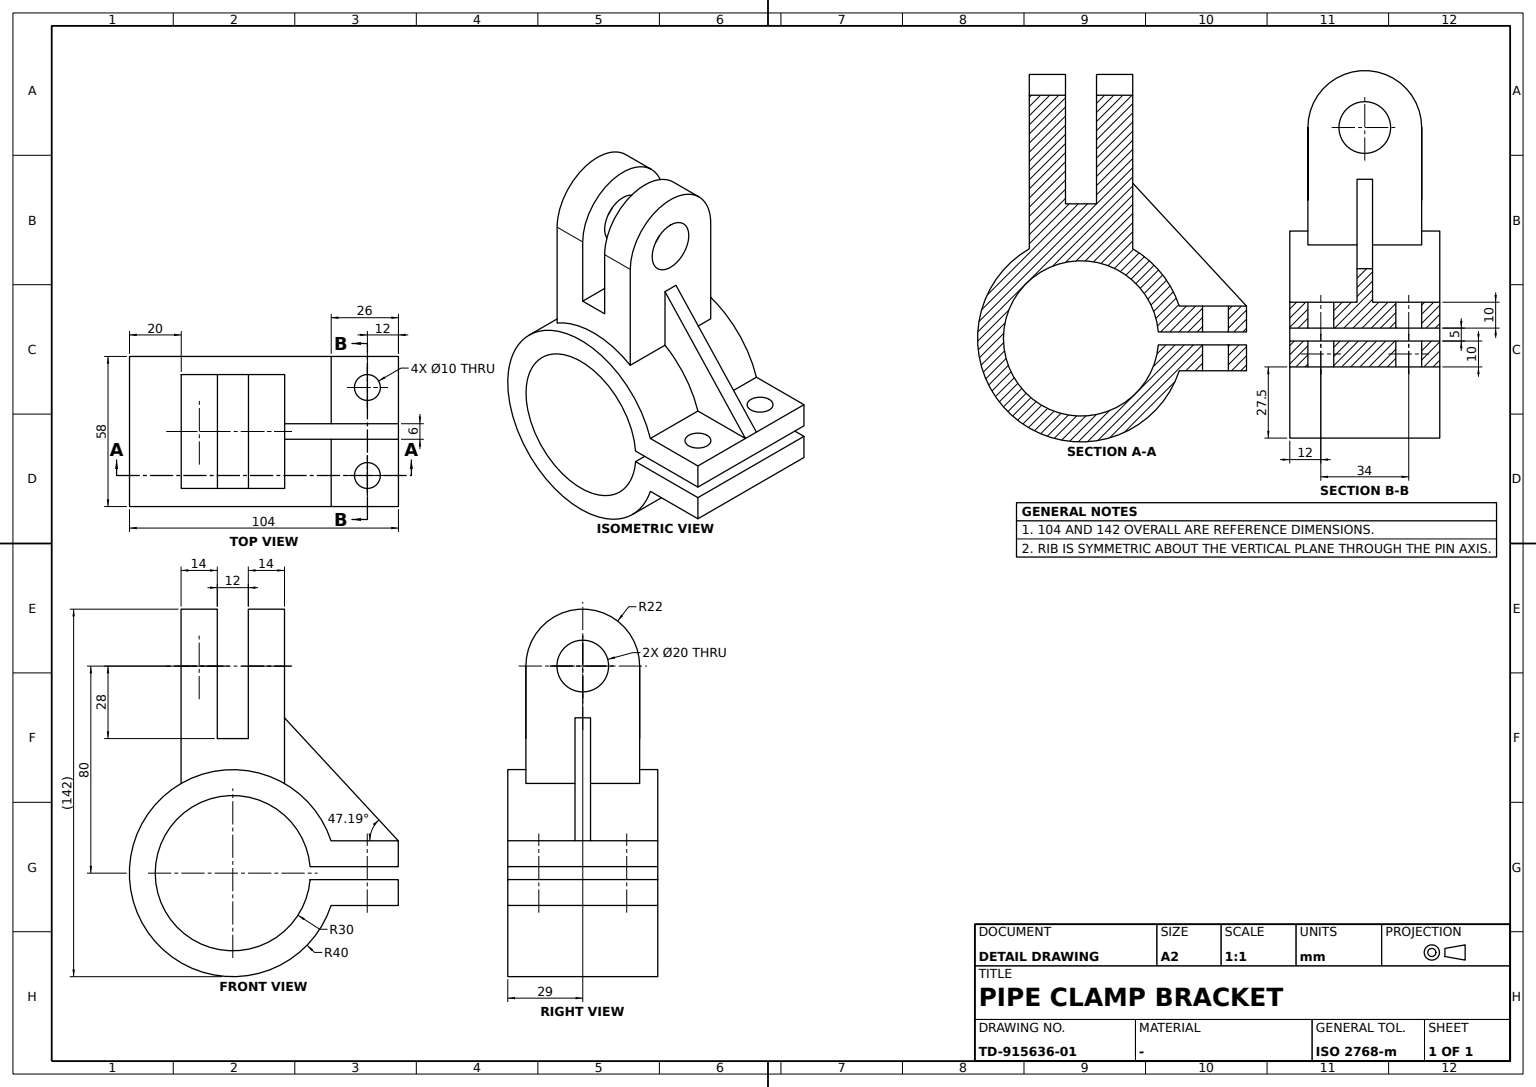
ISO-10303-21;
HEADER;
FILE_DESCRIPTION((''),'2;1');
FILE_NAME('','',(''),(''),'','','');
FILE_SCHEMA(('AUTOMOTIVE_DESIGN'));
ENDSEC;
DATA;
#1=APPLICATION_CONTEXT('');
#2=PRODUCT_CONTEXT('',#1,'mechanical');
#3=PRODUCT('','','',(#2));
#4=PRODUCT_DEFINITION_FORMATION('','',#3);
#5=PRODUCT_DEFINITION_CONTEXT('',#1,'design');
#6=PRODUCT_DEFINITION('','',#4,#5);
#7=PRODUCT_DEFINITION_SHAPE('','',#6);
#8=(LENGTH_UNIT()NAMED_UNIT(*)SI_UNIT(.MILLI.,.METRE.));
#9=(NAMED_UNIT(*)PLANE_ANGLE_UNIT()SI_UNIT($,.RADIAN.));
#10=(NAMED_UNIT(*)SI_UNIT($,.STERADIAN.)SOLID_ANGLE_UNIT());
#11=UNCERTAINTY_MEASURE_WITH_UNIT(LENGTH_MEASURE(0.005),#8,'distance_accuracy_value','');
#12=(GEOMETRIC_REPRESENTATION_CONTEXT(3)GLOBAL_UNCERTAINTY_ASSIGNED_CONTEXT((#11))GLOBAL_UNIT_ASSIGNED_CONTEXT((#8,#9,#10))REPRESENTATION_CONTEXT('',''));
#13=CARTESIAN_POINT('',(-12.,51.99671,2.5));
#14=VERTEX_POINT('',#13);
#15=CARTESIAN_POINT('',(-17.,51.99671,2.5));
#16=DIRECTION('',(0.,0.,1.));
#17=DIRECTION('',(1.,0.,0.));
#18=AXIS2_PLACEMENT_3D('',#15,#16,#17);
#19=CIRCLE('',#18,5.);
#20=EDGE_CURVE('',#14,#14,#19,.T.);
#21=ORIENTED_EDGE('',*,*,#20,.F.);
#22=EDGE_LOOP('',(#21));
#23=FACE_BOUND('',#22,.T.);
#24=CARTESIAN_POINT('',(-22.,51.99671,12.5));
#25=VERTEX_POINT('',#24);
#26=CARTESIAN_POINT('',(-17.,51.99671,12.5));
#27=DIRECTION('',(0.,0.,-1.));
#28=DIRECTION('',(-1.,0.,0.));
#29=AXIS2_PLACEMENT_3D('',#26,#27,#28);
#30=CIRCLE('',#29,5.);
#31=EDGE_CURVE('',#25,#25,#30,.F.);
#32=ORIENTED_EDGE('',*,*,#31,.T.);
#33=EDGE_LOOP('',(#32));
#34=FACE_BOUND('',#33,.T.);
#35=CARTESIAN_POINT('',(-17.,51.99671,-14.41));
#36=DIRECTION('',(0.,-1.,0.));
#37=AXIS2_PLACEMENT_3D('',#35,#16,#36);
#38=CYLINDRICAL_SURFACE('',#37,5.);
#39=ADVANCED_FACE('',(#23,#34),#38,.F.);
#40=CARTESIAN_POINT('',(-3.,63.99671,12.5));
#41=VERTEX_POINT('',#40);
#42=CARTESIAN_POINT('',(3.,63.99671,12.5));
#43=VERTEX_POINT('',#42);
#44=CARTESIAN_POINT('',(0.,63.99671,12.5));
#45=VECTOR('',#17,1000.);
#46=LINE('',#44,#45);
#47=EDGE_CURVE('',#41,#43,#46,.T.);
#48=ORIENTED_EDGE('',*,*,#47,.F.);
#49=CARTESIAN_POINT('',(-3.,20.,60.));
#50=VERTEX_POINT('',#49);
#51=CARTESIAN_POINT('',(-3.,40.67682,37.676764));
#52=DIRECTION('',(0.,0.679534661,-0.733643404));
#53=VECTOR('',#52,1000.);
#54=LINE('',#51,#53);
#55=EDGE_CURVE('',#50,#41,#54,.T.);
#56=ORIENTED_EDGE('',*,*,#55,.F.);
#57=CARTESIAN_POINT('',(3.,20.,60.));
#58=VERTEX_POINT('',#57);
#59=CARTESIAN_POINT('',(0.,20.,60.));
#60=LINE('',#59,#45);
#61=EDGE_CURVE('',#50,#58,#60,.T.);
#62=ORIENTED_EDGE('',*,*,#61,.T.);
#63=CARTESIAN_POINT('',(3.,40.67682,37.676764));
#64=LINE('',#63,#53);
#65=EDGE_CURVE('',#58,#43,#64,.T.);
#66=ORIENTED_EDGE('',*,*,#65,.T.);
#67=EDGE_LOOP('',(#48,#56,#62,#66));
#68=FACE_BOUND('',#67,.T.);
#69=DIRECTION('',(0.,-0.733643404,-0.679534661));
#70=AXIS2_PLACEMENT_3D('',#59,#69,#52);
#71=PLANE('',#70);
#72=ADVANCED_FACE('',(#68),#71,.F.);
#73=CARTESIAN_POINT('',(22.,-20.,80.));
#74=VERTEX_POINT('',#73);
#75=CARTESIAN_POINT('',(22.,-6.,80.));
#76=VERTEX_POINT('',#75);
#77=CARTESIAN_POINT('',(22.,13.,80.));
#78=DIRECTION('',(0.,1.,0.));
#79=VECTOR('',#78,1000.);
#80=LINE('',#77,#79);
#81=EDGE_CURVE('',#74,#76,#80,.T.);
#82=ORIENTED_EDGE('',*,*,#81,.T.);
#83=CARTESIAN_POINT('',(-22.,-6.,80.));
#84=VERTEX_POINT('',#83);
#85=CARTESIAN_POINT('',(0.,-6.,80.));
#86=AXIS2_PLACEMENT_3D('',#85,#36,#27);
#87=CIRCLE('',#86,22.);
#88=EDGE_CURVE('',#84,#76,#87,.F.);
#89=ORIENTED_EDGE('',*,*,#88,.F.);
#90=CARTESIAN_POINT('',(-22.,-20.,80.));
#91=VERTEX_POINT('',#90);
#92=CARTESIAN_POINT('',(-22.,13.,80.));
#93=LINE('',#92,#79);
#94=EDGE_CURVE('',#91,#84,#93,.T.);
#95=ORIENTED_EDGE('',*,*,#94,.F.);
#96=CARTESIAN_POINT('',(0.,-20.,80.));
#97=AXIS2_PLACEMENT_3D('',#96,#78,#16);
#98=CIRCLE('',#97,22.);
#99=EDGE_CURVE('',#91,#74,#98,.T.);
#100=ORIENTED_EDGE('',*,*,#99,.T.);
#101=EDGE_LOOP('',(#82,#89,#95,#100));
#102=FACE_BOUND('',#101,.T.);
#103=CARTESIAN_POINT('',(0.,13.,80.));
#104=AXIS2_PLACEMENT_3D('',#103,#78,#28);
#105=CYLINDRICAL_SURFACE('',#104,22.);
#106=ADVANCED_FACE('',(#102),#105,.T.);
#107=CARTESIAN_POINT('',(0.,20.,70.));
#108=VERTEX_POINT('',#107);
#109=CARTESIAN_POINT('',(0.,20.,80.));
#110=AXIS2_PLACEMENT_3D('',#109,#36,#27);
#111=CIRCLE('',#110,10.);
#112=EDGE_CURVE('',#108,#108,#111,.F.);
#113=ORIENTED_EDGE('',*,*,#112,.T.);
#114=EDGE_LOOP('',(#113));
#115=FACE_BOUND('',#114,.T.);
#116=CARTESIAN_POINT('',(0.,6.,90.));
#117=VERTEX_POINT('',#116);
#118=CARTESIAN_POINT('',(0.,6.,80.));
#119=AXIS2_PLACEMENT_3D('',#118,#78,#16);
#120=CIRCLE('',#119,10.);
#121=EDGE_CURVE('',#117,#117,#120,.T.);
#122=ORIENTED_EDGE('',*,*,#121,.F.);
#123=EDGE_LOOP('',(#122));
#124=FACE_BOUND('',#123,.T.);
#125=CYLINDRICAL_SURFACE('',#104,10.);
#126=ADVANCED_FACE('',(#115,#124),#125,.F.);
#127=CARTESIAN_POINT('',(3.,37.99671,12.5));
#128=VERTEX_POINT('',#127);
#129=CARTESIAN_POINT('',(3.,20.,34.641016));
#130=VERTEX_POINT('',#129);
#131=CARTESIAN_POINT('',(3.,0.,0.));
#132=AXIS2_PLACEMENT_3D('',#131,#17,#27);
#133=CIRCLE('',#132,40.);
#134=EDGE_CURVE('',#128,#130,#133,.T.);
#135=ORIENTED_EDGE('',*,*,#134,.F.);
#136=VECTOR('',#36,1000.);
#137=LINE('',#127,#136);
#138=EDGE_CURVE('',#43,#128,#137,.T.);
#139=ORIENTED_EDGE('',*,*,#138,.F.);
#140=ORIENTED_EDGE('',*,*,#65,.F.);
#141=CARTESIAN_POINT('',(3.,20.,0.));
#142=VECTOR('',#27,1000.);
#143=LINE('',#141,#142);
#144=EDGE_CURVE('',#58,#130,#143,.T.);
#145=ORIENTED_EDGE('',*,*,#144,.T.);
#146=EDGE_LOOP('',(#135,#139,#140,#145));
#147=FACE_BOUND('',#146,.T.);
#148=AXIS2_PLACEMENT_3D('',#131,#17,#78);
#149=PLANE('',#148);
#150=ADVANCED_FACE('',(#147),#149,.T.);
#151=CARTESIAN_POINT('',(-22.,20.,80.));
#152=VERTEX_POINT('',#151);
#153=CARTESIAN_POINT('',(22.,20.,80.));
#154=VERTEX_POINT('',#153);
#155=CIRCLE('',#110,22.);
#156=EDGE_CURVE('',#152,#154,#155,.F.);
#157=ORIENTED_EDGE('',*,*,#156,.F.);
#158=CARTESIAN_POINT('',(-22.,6.,80.));
#159=VERTEX_POINT('',#158);
#160=EDGE_CURVE('',#152,#159,#93,.F.);
#161=ORIENTED_EDGE('',*,*,#160,.T.);
#162=CARTESIAN_POINT('',(22.,6.,80.));
#163=VERTEX_POINT('',#162);
#164=CIRCLE('',#119,22.);
#165=EDGE_CURVE('',#159,#163,#164,.T.);
#166=ORIENTED_EDGE('',*,*,#165,.T.);
#167=EDGE_CURVE('',#154,#163,#80,.F.);
#168=ORIENTED_EDGE('',*,*,#167,.F.);
#169=EDGE_LOOP('',(#157,#161,#166,#168));
#170=FACE_BOUND('',#169,.T.);
#171=ADVANCED_FACE('',(#170),#105,.T.);
#172=CARTESIAN_POINT('',(-22.,51.99671,-2.5));
#173=VERTEX_POINT('',#172);
#174=CARTESIAN_POINT('',(-17.,51.99671,-2.5));
#175=AXIS2_PLACEMENT_3D('',#174,#27,#28);
#176=CIRCLE('',#175,5.);
#177=EDGE_CURVE('',#173,#173,#176,.T.);
#178=ORIENTED_EDGE('',*,*,#177,.T.);
#179=EDGE_LOOP('',(#178));
#180=FACE_BOUND('',#179,.T.);
#181=CARTESIAN_POINT('',(-29.,63.99671,-2.5));
#182=VERTEX_POINT('',#181);
#183=CARTESIAN_POINT('',(29.,63.99671,-2.5));
#184=VERTEX_POINT('',#183);
#185=CARTESIAN_POINT('',(0.,63.99671,-2.5));
#186=LINE('',#185,#45);
#187=EDGE_CURVE('',#182,#184,#186,.T.);
#188=ORIENTED_EDGE('',*,*,#187,.F.);
#189=CARTESIAN_POINT('',(-29.,29.895652,-2.5));
#190=VERTEX_POINT('',#189);
#191=CARTESIAN_POINT('',(-29.,0.,-2.5));
#192=LINE('',#191,#79);
#193=EDGE_CURVE('',#190,#182,#192,.T.);
#194=ORIENTED_EDGE('',*,*,#193,.F.);
#195=CARTESIAN_POINT('',(29.,29.895652,-2.5));
#196=VERTEX_POINT('',#195);
#197=LINE('',#189,#45);
#198=EDGE_CURVE('',#190,#196,#197,.T.);
#199=ORIENTED_EDGE('',*,*,#198,.T.);
#200=CARTESIAN_POINT('',(29.,0.,-2.5));
#201=LINE('',#200,#79);
#202=EDGE_CURVE('',#196,#184,#201,.T.);
#203=ORIENTED_EDGE('',*,*,#202,.T.);
#204=EDGE_LOOP('',(#188,#194,#199,#203));
#205=FACE_BOUND('',#204,.T.);
#206=CARTESIAN_POINT('',(12.,51.99671,-2.5));
#207=VERTEX_POINT('',#206);
#208=CARTESIAN_POINT('',(17.,51.99671,-2.5));
#209=AXIS2_PLACEMENT_3D('',#208,#27,#28);
#210=CIRCLE('',#209,5.);
#211=EDGE_CURVE('',#207,#207,#210,.T.);
#212=ORIENTED_EDGE('',*,*,#211,.T.);
#213=EDGE_LOOP('',(#212));
#214=FACE_BOUND('',#213,.T.);
#215=CARTESIAN_POINT('',(0.,29.895652,-2.5));
#216=AXIS2_PLACEMENT_3D('',#215,#27,#78);
#217=PLANE('',#216);
#218=ADVANCED_FACE('',(#180,#205,#214),#217,.F.);
#219=CARTESIAN_POINT('',(-22.,-20.,34.641016));
#220=VERTEX_POINT('',#219);
#221=LINE('',#219,#142);
#222=EDGE_CURVE('',#91,#220,#221,.T.);
#223=ORIENTED_EDGE('',*,*,#222,.F.);
#224=ORIENTED_EDGE('',*,*,#94,.T.);
#225=CARTESIAN_POINT('',(-22.,-6.,52.));
#226=VERTEX_POINT('',#225);
#227=CARTESIAN_POINT('',(-22.,-6.,0.));
#228=LINE('',#227,#142);
#229=EDGE_CURVE('',#84,#226,#228,.T.);
#230=ORIENTED_EDGE('',*,*,#229,.T.);
#231=CARTESIAN_POINT('',(-22.,6.,52.));
#232=VERTEX_POINT('',#231);
#233=CARTESIAN_POINT('',(-22.,0.,52.));
#234=LINE('',#233,#79);
#235=EDGE_CURVE('',#226,#232,#234,.T.);
#236=ORIENTED_EDGE('',*,*,#235,.T.);
#237=LINE('',#231,#142);
#238=EDGE_CURVE('',#159,#232,#237,.T.);
#239=ORIENTED_EDGE('',*,*,#238,.F.);
#240=ORIENTED_EDGE('',*,*,#160,.F.);
#241=CARTESIAN_POINT('',(-22.,20.,34.641016));
#242=VERTEX_POINT('',#241);
#243=CARTESIAN_POINT('',(-22.,20.,0.));
#244=LINE('',#243,#142);
#245=EDGE_CURVE('',#152,#242,#244,.T.);
#246=ORIENTED_EDGE('',*,*,#245,.T.);
#247=CARTESIAN_POINT('',(-22.,0.,0.));
#248=AXIS2_PLACEMENT_3D('',#247,#17,#27);
#249=CIRCLE('',#248,40.);
#250=EDGE_CURVE('',#242,#220,#249,.T.);
#251=ORIENTED_EDGE('',*,*,#250,.T.);
#252=EDGE_LOOP('',(#223,#224,#230,#236,#239,#240,#246,#251));
#253=FACE_BOUND('',#252,.T.);
#254=AXIS2_PLACEMENT_3D('',#247,#17,#78);
#255=PLANE('',#254);
#256=ADVANCED_FACE('',(#253),#255,.F.);
#257=ORIENTED_EDGE('',*,*,#121,.T.);
#258=EDGE_LOOP('',(#257));
#259=FACE_BOUND('',#258,.T.);
#260=CARTESIAN_POINT('',(22.,6.,52.));
#261=VERTEX_POINT('',#260);
#262=CARTESIAN_POINT('',(0.,6.,52.));
#263=LINE('',#262,#45);
#264=EDGE_CURVE('',#232,#261,#263,.T.);
#265=ORIENTED_EDGE('',*,*,#264,.T.);
#266=LINE('',#260,#142);
#267=EDGE_CURVE('',#163,#261,#266,.T.);
#268=ORIENTED_EDGE('',*,*,#267,.F.);
#269=ORIENTED_EDGE('',*,*,#165,.F.);
#270=ORIENTED_EDGE('',*,*,#238,.T.);
#271=EDGE_LOOP('',(#265,#268,#269,#270));
#272=FACE_BOUND('',#271,.T.);
#273=AXIS2_PLACEMENT_3D('',#262,#78,#16);
#274=PLANE('',#273);
#275=ADVANCED_FACE('',(#259,#272),#274,.F.);
#276=CARTESIAN_POINT('',(22.,-6.,52.));
#277=VERTEX_POINT('',#276);
#278=CARTESIAN_POINT('',(22.,-6.,0.));
#279=LINE('',#278,#142);
#280=EDGE_CURVE('',#76,#277,#279,.T.);
#281=ORIENTED_EDGE('',*,*,#280,.T.);
#282=CARTESIAN_POINT('',(0.,-6.,52.));
#283=LINE('',#282,#45);
#284=EDGE_CURVE('',#226,#277,#283,.T.);
#285=ORIENTED_EDGE('',*,*,#284,.F.);
#286=ORIENTED_EDGE('',*,*,#229,.F.);
#287=ORIENTED_EDGE('',*,*,#88,.T.);
#288=EDGE_LOOP('',(#281,#285,#286,#287));
#289=FACE_BOUND('',#288,.T.);
#290=CARTESIAN_POINT('',(0.,-6.,70.));
#291=VERTEX_POINT('',#290);
#292=CIRCLE('',#86,10.);
#293=EDGE_CURVE('',#291,#291,#292,.F.);
#294=ORIENTED_EDGE('',*,*,#293,.F.);
#295=EDGE_LOOP('',(#294));
#296=FACE_BOUND('',#295,.T.);
#297=PLANE('',#86);
#298=ADVANCED_FACE('',(#289,#296),#297,.F.);
#299=CARTESIAN_POINT('',(-29.,63.99671,12.5));
#300=VERTEX_POINT('',#299);
#301=CARTESIAN_POINT('',(-29.,63.99671,2.5));
#302=VERTEX_POINT('',#301);
#303=CARTESIAN_POINT('',(-29.,63.99671,0.));
#304=LINE('',#303,#142);
#305=EDGE_CURVE('',#300,#302,#304,.T.);
#306=ORIENTED_EDGE('',*,*,#305,.F.);
#307=EDGE_CURVE('',#300,#41,#46,.T.);
#308=ORIENTED_EDGE('',*,*,#307,.T.);
#309=ORIENTED_EDGE('',*,*,#47,.T.);
#310=CARTESIAN_POINT('',(29.,63.99671,12.5));
#311=VERTEX_POINT('',#310);
#312=EDGE_CURVE('',#43,#311,#46,.T.);
#313=ORIENTED_EDGE('',*,*,#312,.T.);
#314=CARTESIAN_POINT('',(29.,63.99671,2.5));
#315=VERTEX_POINT('',#314);
#316=CARTESIAN_POINT('',(29.,63.99671,0.));
#317=LINE('',#316,#142);
#318=EDGE_CURVE('',#311,#315,#317,.T.);
#319=ORIENTED_EDGE('',*,*,#318,.T.);
#320=CARTESIAN_POINT('',(0.,63.99671,2.5));
#321=LINE('',#320,#45);
#322=EDGE_CURVE('',#302,#315,#321,.T.);
#323=ORIENTED_EDGE('',*,*,#322,.F.);
#324=EDGE_LOOP('',(#306,#308,#309,#313,#319,#323));
#325=FACE_BOUND('',#324,.T.);
#326=AXIS2_PLACEMENT_3D('',#185,#36,#27);
#327=PLANE('',#326);
#328=ADVANCED_FACE('',(#325),#327,.F.);
#329=ORIENTED_EDGE('',*,*,#99,.F.);
#330=ORIENTED_EDGE('',*,*,#222,.T.);
#331=CARTESIAN_POINT('',(22.,-20.,34.641016));
#332=VERTEX_POINT('',#331);
#333=LINE('',#219,#45);
#334=EDGE_CURVE('',#220,#332,#333,.T.);
#335=ORIENTED_EDGE('',*,*,#334,.T.);
#336=LINE('',#331,#142);
#337=EDGE_CURVE('',#74,#332,#336,.T.);
#338=ORIENTED_EDGE('',*,*,#337,.F.);
#339=EDGE_LOOP('',(#329,#330,#335,#338));
#340=FACE_BOUND('',#339,.T.);
#341=CARTESIAN_POINT('',(0.,-20.,90.));
#342=VERTEX_POINT('',#341);
#343=CIRCLE('',#97,10.);
#344=EDGE_CURVE('',#342,#342,#343,.T.);
#345=ORIENTED_EDGE('',*,*,#344,.T.);
#346=EDGE_LOOP('',(#345));
#347=FACE_BOUND('',#346,.T.);
#348=CARTESIAN_POINT('',(0.,-20.,34.641016));
#349=AXIS2_PLACEMENT_3D('',#348,#78,#16);
#350=PLANE('',#349);
#351=ADVANCED_FACE('',(#340,#347),#350,.F.);
#352=CARTESIAN_POINT('',(22.,0.,52.));
#353=LINE('',#352,#79);
#354=EDGE_CURVE('',#277,#261,#353,.T.);
#355=ORIENTED_EDGE('',*,*,#354,.T.);
#356=ORIENTED_EDGE('',*,*,#264,.F.);
#357=ORIENTED_EDGE('',*,*,#235,.F.);
#358=ORIENTED_EDGE('',*,*,#284,.T.);
#359=EDGE_LOOP('',(#355,#356,#357,#358));
#360=FACE_BOUND('',#359,.T.);
#361=AXIS2_PLACEMENT_3D('',#282,#27,#78);
#362=PLANE('',#361);
#363=ADVANCED_FACE('',(#360),#362,.F.);
#364=ORIENTED_EDGE('',*,*,#112,.F.);
#365=EDGE_LOOP('',(#364));
#366=FACE_BOUND('',#365,.T.);
#367=CARTESIAN_POINT('',(22.,20.,34.641016));
#368=VERTEX_POINT('',#367);
#369=CARTESIAN_POINT('',(22.,20.,0.));
#370=LINE('',#369,#142);
#371=EDGE_CURVE('',#154,#368,#370,.T.);
#372=ORIENTED_EDGE('',*,*,#371,.T.);
#373=LINE('',#129,#45);
#374=EDGE_CURVE('',#130,#368,#373,.T.);
#375=ORIENTED_EDGE('',*,*,#374,.F.);
#376=ORIENTED_EDGE('',*,*,#144,.F.);
#377=ORIENTED_EDGE('',*,*,#61,.F.);
#378=CARTESIAN_POINT('',(-3.,20.,34.641016));
#379=VERTEX_POINT('',#378);
#380=CARTESIAN_POINT('',(-3.,20.,0.));
#381=LINE('',#380,#142);
#382=EDGE_CURVE('',#50,#379,#381,.T.);
#383=ORIENTED_EDGE('',*,*,#382,.T.);
#384=LINE('',#241,#45);
#385=EDGE_CURVE('',#242,#379,#384,.T.);
#386=ORIENTED_EDGE('',*,*,#385,.F.);
#387=ORIENTED_EDGE('',*,*,#245,.F.);
#388=ORIENTED_EDGE('',*,*,#156,.T.);
#389=EDGE_LOOP('',(#372,#375,#376,#377,#383,#386,#387,#388));
#390=FACE_BOUND('',#389,.T.);
#391=PLANE('',#110);
#392=ADVANCED_FACE('',(#366,#390),#391,.F.);
#393=CARTESIAN_POINT('',(22.,0.,0.));
#394=AXIS2_PLACEMENT_3D('',#393,#17,#27);
#395=CIRCLE('',#394,40.);
#396=EDGE_CURVE('',#368,#332,#395,.T.);
#397=ORIENTED_EDGE('',*,*,#396,.F.);
#398=ORIENTED_EDGE('',*,*,#371,.F.);
#399=ORIENTED_EDGE('',*,*,#167,.T.);
#400=ORIENTED_EDGE('',*,*,#267,.T.);
#401=ORIENTED_EDGE('',*,*,#354,.F.);
#402=ORIENTED_EDGE('',*,*,#280,.F.);
#403=ORIENTED_EDGE('',*,*,#81,.F.);
#404=ORIENTED_EDGE('',*,*,#337,.T.);
#405=EDGE_LOOP('',(#397,#398,#399,#400,#401,#402,#403,#404));
#406=FACE_BOUND('',#405,.T.);
#407=AXIS2_PLACEMENT_3D('',#393,#17,#78);
#408=PLANE('',#407);
#409=ADVANCED_FACE('',(#406),#408,.T.);
#410=CARTESIAN_POINT('',(29.,37.99671,12.5));
#411=VERTEX_POINT('',#410);
#412=LINE('',#127,#45);
#413=EDGE_CURVE('',#128,#411,#412,.T.);
#414=ORIENTED_EDGE('',*,*,#413,.T.);
#415=CARTESIAN_POINT('',(29.,0.,12.5));
#416=LINE('',#415,#79);
#417=EDGE_CURVE('',#411,#311,#416,.T.);
#418=ORIENTED_EDGE('',*,*,#417,.T.);
#419=ORIENTED_EDGE('',*,*,#312,.F.);
#420=ORIENTED_EDGE('',*,*,#138,.T.);
#421=EDGE_LOOP('',(#414,#418,#419,#420));
#422=FACE_BOUND('',#421,.T.);
#423=CARTESIAN_POINT('',(12.,51.99671,12.5));
#424=VERTEX_POINT('',#423);
#425=CARTESIAN_POINT('',(17.,51.99671,12.5));
#426=AXIS2_PLACEMENT_3D('',#425,#27,#28);
#427=CIRCLE('',#426,5.);
#428=EDGE_CURVE('',#424,#424,#427,.F.);
#429=ORIENTED_EDGE('',*,*,#428,.F.);
#430=EDGE_LOOP('',(#429));
#431=FACE_BOUND('',#430,.T.);
#432=CARTESIAN_POINT('',(0.,37.99671,12.5));
#433=AXIS2_PLACEMENT_3D('',#432,#27,#78);
#434=PLANE('',#433);
#435=ADVANCED_FACE('',(#422,#431),#434,.F.);
#436=ORIENTED_EDGE('',*,*,#413,.F.);
#437=ORIENTED_EDGE('',*,*,#134,.T.);
#438=ORIENTED_EDGE('',*,*,#374,.T.);
#439=ORIENTED_EDGE('',*,*,#396,.T.);
#440=ORIENTED_EDGE('',*,*,#334,.F.);
#441=ORIENTED_EDGE('',*,*,#250,.F.);
#442=ORIENTED_EDGE('',*,*,#385,.T.);
#443=CARTESIAN_POINT('',(-3.,37.99671,12.5));
#444=VERTEX_POINT('',#443);
#445=CARTESIAN_POINT('',(-3.,0.,0.));
#446=AXIS2_PLACEMENT_3D('',#445,#17,#27);
#447=CIRCLE('',#446,40.);
#448=EDGE_CURVE('',#444,#379,#447,.T.);
#449=ORIENTED_EDGE('',*,*,#448,.F.);
#450=CARTESIAN_POINT('',(-29.,37.99671,12.5));
#451=VERTEX_POINT('',#450);
#452=LINE('',#450,#45);
#453=EDGE_CURVE('',#451,#444,#452,.T.);
#454=ORIENTED_EDGE('',*,*,#453,.F.);
#455=CARTESIAN_POINT('',(-29.,37.99671,-12.5));
#456=VERTEX_POINT('',#455);
#457=CARTESIAN_POINT('',(-29.,0.,0.));
#458=AXIS2_PLACEMENT_3D('',#457,#17,#27);
#459=CIRCLE('',#458,40.);
#460=EDGE_CURVE('',#451,#456,#459,.T.);
#461=ORIENTED_EDGE('',*,*,#460,.T.);
#462=CARTESIAN_POINT('',(29.,37.99671,-12.5));
#463=VERTEX_POINT('',#462);
#464=LINE('',#455,#45);
#465=EDGE_CURVE('',#456,#463,#464,.T.);
#466=ORIENTED_EDGE('',*,*,#465,.T.);
#467=CARTESIAN_POINT('',(29.,0.,0.));
#468=AXIS2_PLACEMENT_3D('',#467,#17,#27);
#469=CIRCLE('',#468,40.);
#470=EDGE_CURVE('',#411,#463,#469,.T.);
#471=ORIENTED_EDGE('',*,*,#470,.F.);
#472=EDGE_LOOP('',(#436,#437,#438,#439,#440,#441,#442,#449,#454,#461,#466,#471));
#473=FACE_BOUND('',#472,.T.);
#474=CARTESIAN_POINT('',(0.,0.,0.));
#475=AXIS2_PLACEMENT_3D('',#474,#17,#78);
#476=CYLINDRICAL_SURFACE('',#475,40.);
#477=ADVANCED_FACE('',(#473),#476,.T.);
#478=CARTESIAN_POINT('',(-29.,29.895652,2.5));
#479=VERTEX_POINT('',#478);
#480=CARTESIAN_POINT('',(29.,29.895652,2.5));
#481=VERTEX_POINT('',#480);
#482=LINE('',#478,#45);
#483=EDGE_CURVE('',#479,#481,#482,.T.);
#484=ORIENTED_EDGE('',*,*,#483,.F.);
#485=CARTESIAN_POINT('',(-29.,0.,2.5));
#486=LINE('',#485,#136);
#487=EDGE_CURVE('',#302,#479,#486,.T.);
#488=ORIENTED_EDGE('',*,*,#487,.F.);
#489=ORIENTED_EDGE('',*,*,#322,.T.);
#490=CARTESIAN_POINT('',(29.,0.,2.5));
#491=LINE('',#490,#136);
#492=EDGE_CURVE('',#315,#481,#491,.T.);
#493=ORIENTED_EDGE('',*,*,#492,.T.);
#494=EDGE_LOOP('',(#484,#488,#489,#493));
#495=FACE_BOUND('',#494,.T.);
#496=CARTESIAN_POINT('',(22.,51.99671,2.5));
#497=VERTEX_POINT('',#496);
#498=CARTESIAN_POINT('',(17.,51.99671,2.5));
#499=AXIS2_PLACEMENT_3D('',#498,#16,#17);
#500=CIRCLE('',#499,5.);
#501=EDGE_CURVE('',#497,#497,#500,.T.);
#502=ORIENTED_EDGE('',*,*,#501,.T.);
#503=EDGE_LOOP('',(#502));
#504=FACE_BOUND('',#503,.T.);
#505=ORIENTED_EDGE('',*,*,#20,.T.);
#506=EDGE_LOOP('',(#505));
#507=FACE_BOUND('',#506,.T.);
#508=AXIS2_PLACEMENT_3D('',#320,#16,#36);
#509=PLANE('',#508);
#510=ADVANCED_FACE('',(#495,#504,#507),#509,.F.);
#511=CARTESIAN_POINT('',(-12.,51.99671,-12.5));
#512=VERTEX_POINT('',#511);
#513=CARTESIAN_POINT('',(-17.,51.99671,-12.5));
#514=AXIS2_PLACEMENT_3D('',#513,#16,#17);
#515=CIRCLE('',#514,5.);
#516=EDGE_CURVE('',#512,#512,#515,.T.);
#517=ORIENTED_EDGE('',*,*,#516,.T.);
#518=EDGE_LOOP('',(#517));
#519=FACE_BOUND('',#518,.T.);
#520=CARTESIAN_POINT('',(22.,51.99671,-12.5));
#521=VERTEX_POINT('',#520);
#522=CARTESIAN_POINT('',(17.,51.99671,-12.5));
#523=AXIS2_PLACEMENT_3D('',#522,#16,#17);
#524=CIRCLE('',#523,5.);
#525=EDGE_CURVE('',#521,#521,#524,.T.);
#526=ORIENTED_EDGE('',*,*,#525,.T.);
#527=EDGE_LOOP('',(#526));
#528=FACE_BOUND('',#527,.T.);
#529=CARTESIAN_POINT('',(-29.,63.99671,-12.5));
#530=VERTEX_POINT('',#529);
#531=CARTESIAN_POINT('',(29.,63.99671,-12.5));
#532=VERTEX_POINT('',#531);
#533=CARTESIAN_POINT('',(0.,63.99671,-12.5));
#534=LINE('',#533,#45);
#535=EDGE_CURVE('',#530,#532,#534,.T.);
#536=ORIENTED_EDGE('',*,*,#535,.T.);
#537=CARTESIAN_POINT('',(29.,0.,-12.5));
#538=LINE('',#537,#136);
#539=EDGE_CURVE('',#532,#463,#538,.T.);
#540=ORIENTED_EDGE('',*,*,#539,.T.);
#541=ORIENTED_EDGE('',*,*,#465,.F.);
#542=CARTESIAN_POINT('',(-29.,0.,-12.5));
#543=LINE('',#542,#136);
#544=EDGE_CURVE('',#530,#456,#543,.T.);
#545=ORIENTED_EDGE('',*,*,#544,.F.);
#546=EDGE_LOOP('',(#536,#540,#541,#545));
#547=FACE_BOUND('',#546,.T.);
#548=AXIS2_PLACEMENT_3D('',#533,#16,#36);
#549=PLANE('',#548);
#550=ADVANCED_FACE('',(#519,#528,#547),#549,.F.);
#551=ORIENTED_EDGE('',*,*,#177,.F.);
#552=EDGE_LOOP('',(#551));
#553=FACE_BOUND('',#552,.T.);
#554=ORIENTED_EDGE('',*,*,#516,.F.);
#555=EDGE_LOOP('',(#554));
#556=FACE_BOUND('',#555,.T.);
#557=ADVANCED_FACE('',(#553,#556),#38,.F.);
#558=ORIENTED_EDGE('',*,*,#453,.T.);
#559=LINE('',#443,#136);
#560=EDGE_CURVE('',#41,#444,#559,.T.);
#561=ORIENTED_EDGE('',*,*,#560,.F.);
#562=ORIENTED_EDGE('',*,*,#307,.F.);
#563=CARTESIAN_POINT('',(-29.,0.,12.5));
#564=LINE('',#563,#79);
#565=EDGE_CURVE('',#451,#300,#564,.T.);
#566=ORIENTED_EDGE('',*,*,#565,.F.);
#567=EDGE_LOOP('',(#558,#561,#562,#566));
#568=FACE_BOUND('',#567,.T.);
#569=ORIENTED_EDGE('',*,*,#31,.F.);
#570=EDGE_LOOP('',(#569));
#571=FACE_BOUND('',#570,.T.);
#572=ADVANCED_FACE('',(#568,#571),#434,.F.);
#573=ORIENTED_EDGE('',*,*,#428,.T.);
#574=EDGE_LOOP('',(#573));
#575=FACE_BOUND('',#574,.T.);
#576=ORIENTED_EDGE('',*,*,#501,.F.);
#577=EDGE_LOOP('',(#576));
#578=FACE_BOUND('',#577,.T.);
#579=CARTESIAN_POINT('',(17.,51.99671,-14.41));
#580=AXIS2_PLACEMENT_3D('',#579,#16,#36);
#581=CYLINDRICAL_SURFACE('',#580,5.);
#582=ADVANCED_FACE('',(#575,#578),#581,.F.);
#583=ORIENTED_EDGE('',*,*,#293,.T.);
#584=EDGE_LOOP('',(#583));
#585=FACE_BOUND('',#584,.T.);
#586=ORIENTED_EDGE('',*,*,#344,.F.);
#587=EDGE_LOOP('',(#586));
#588=FACE_BOUND('',#587,.T.);
#589=ADVANCED_FACE('',(#585,#588),#125,.F.);
#590=ORIENTED_EDGE('',*,*,#198,.F.);
#591=CIRCLE('',#458,30.);
#592=EDGE_CURVE('',#479,#190,#591,.T.);
#593=ORIENTED_EDGE('',*,*,#592,.F.);
#594=ORIENTED_EDGE('',*,*,#483,.T.);
#595=CIRCLE('',#468,30.);
#596=EDGE_CURVE('',#481,#196,#595,.T.);
#597=ORIENTED_EDGE('',*,*,#596,.T.);
#598=EDGE_LOOP('',(#590,#593,#594,#597));
#599=FACE_BOUND('',#598,.T.);
#600=CYLINDRICAL_SURFACE('',#475,30.);
#601=ADVANCED_FACE('',(#599),#600,.F.);
#602=ORIENTED_EDGE('',*,*,#211,.F.);
#603=EDGE_LOOP('',(#602));
#604=FACE_BOUND('',#603,.T.);
#605=ORIENTED_EDGE('',*,*,#525,.F.);
#606=EDGE_LOOP('',(#605));
#607=FACE_BOUND('',#606,.T.);
#608=ADVANCED_FACE('',(#604,#607),#581,.F.);
#609=ORIENTED_EDGE('',*,*,#460,.F.);
#610=ORIENTED_EDGE('',*,*,#565,.T.);
#611=ORIENTED_EDGE('',*,*,#305,.T.);
#612=ORIENTED_EDGE('',*,*,#487,.T.);
#613=ORIENTED_EDGE('',*,*,#592,.T.);
#614=ORIENTED_EDGE('',*,*,#193,.T.);
#615=EDGE_CURVE('',#182,#530,#304,.T.);
#616=ORIENTED_EDGE('',*,*,#615,.T.);
#617=ORIENTED_EDGE('',*,*,#544,.T.);
#618=EDGE_LOOP('',(#609,#610,#611,#612,#613,#614,#616,#617));
#619=FACE_BOUND('',#618,.T.);
#620=AXIS2_PLACEMENT_3D('',#457,#17,#78);
#621=PLANE('',#620);
#622=ADVANCED_FACE('',(#619),#621,.F.);
#623=ORIENTED_EDGE('',*,*,#539,.F.);
#624=EDGE_CURVE('',#184,#532,#317,.T.);
#625=ORIENTED_EDGE('',*,*,#624,.F.);
#626=ORIENTED_EDGE('',*,*,#202,.F.);
#627=ORIENTED_EDGE('',*,*,#596,.F.);
#628=ORIENTED_EDGE('',*,*,#492,.F.);
#629=ORIENTED_EDGE('',*,*,#318,.F.);
#630=ORIENTED_EDGE('',*,*,#417,.F.);
#631=ORIENTED_EDGE('',*,*,#470,.T.);
#632=EDGE_LOOP('',(#623,#625,#626,#627,#628,#629,#630,#631));
#633=FACE_BOUND('',#632,.T.);
#634=AXIS2_PLACEMENT_3D('',#467,#17,#78);
#635=PLANE('',#634);
#636=ADVANCED_FACE('',(#633),#635,.T.);
#637=ORIENTED_EDGE('',*,*,#560,.T.);
#638=ORIENTED_EDGE('',*,*,#448,.T.);
#639=ORIENTED_EDGE('',*,*,#382,.F.);
#640=ORIENTED_EDGE('',*,*,#55,.T.);
#641=EDGE_LOOP('',(#637,#638,#639,#640));
#642=FACE_BOUND('',#641,.T.);
#643=AXIS2_PLACEMENT_3D('',#445,#17,#78);
#644=PLANE('',#643);
#645=ADVANCED_FACE('',(#642),#644,.F.);
#646=ORIENTED_EDGE('',*,*,#624,.T.);
#647=ORIENTED_EDGE('',*,*,#535,.F.);
#648=ORIENTED_EDGE('',*,*,#615,.F.);
#649=ORIENTED_EDGE('',*,*,#187,.T.);
#650=EDGE_LOOP('',(#646,#647,#648,#649));
#651=FACE_BOUND('',#650,.T.);
#652=ADVANCED_FACE('',(#651),#327,.F.);
#653=CLOSED_SHELL('',(#39,#72,#106,#126,#150,#171,#218,#256,#275,#298,#328,#351,#363,#392,#409,#435,#477,#510,#550,#557,#572,#582,#589,#601,#608,#622,#636,#645,#652));
#654=MANIFOLD_SOLID_BREP('',#653);
#655=ADVANCED_BREP_SHAPE_REPRESENTATION('',(#654),#12);
#656=SHAPE_DEFINITION_REPRESENTATION(#7,#655);
ENDSEC;
END-ISO-10303-21;
